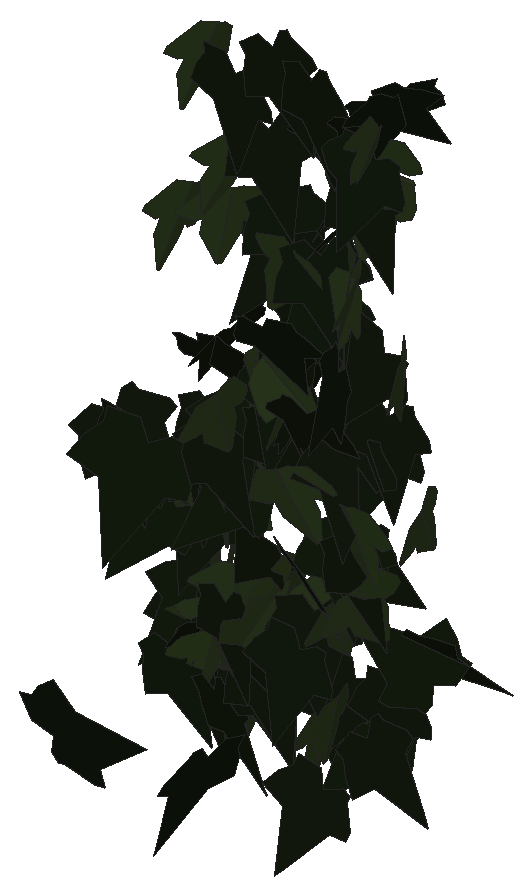
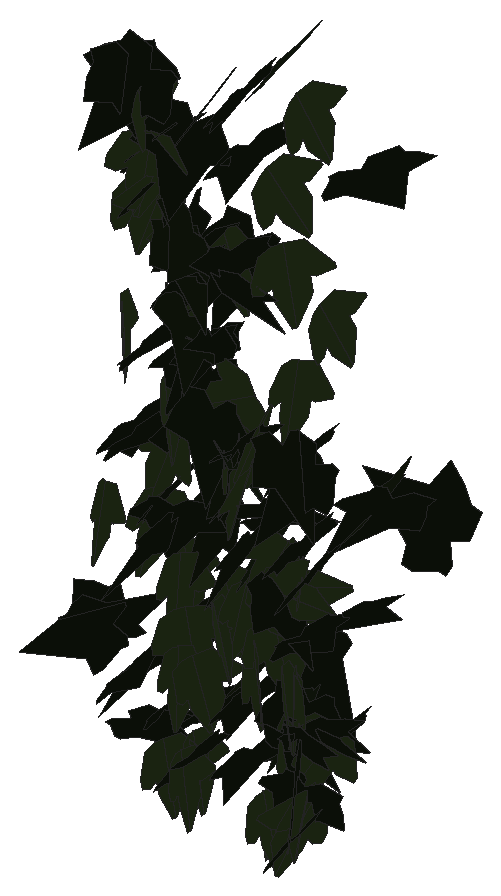
# SketchUp Ruby script. Lengths in inches.
U = 1.inch
M = Sketchup.active_model
def pt(a) = Geom::Point3d.new(a.map { |v| v * U })
def face(e, loops, mat)
  f = e.add_face(loops[0].map { |a| pt(a) })
  loops[1..].each { |l| e.add_face(l.map { |a| pt(a) }).erase! }
  f.material = f.back_material = mat if mat
  f
end
# faces: each face lists its corners as indices into pts; further lists are holes
def faces(e, pts, list, mat = nil) = list.each { |f| face(e, (f[0].is_a?(Array) ? f : [f]).map { |l| l.map { |i| pts[i] } }, mat) }
# xy, xz, yz: faces in a plane at the given z, y or x. An outline is a flat list of corners, or four numbers for a rectangle; further outlines are holes
def ring(l) = l.size == 4 ? [[l[0], l[1]], [l[2], l[1]], [l[2], l[3]], [l[0], l[3]]] : l.each_slice(2).to_a
def flat(e, list, mat, &to3) = list.each { |f| face(e, (f[0].is_a?(Array) ? f : [f]).map { |l| ring(l).map { |u, v| to3.(u, v) } }, mat) }
def xy(e, z, list, mat = nil) = flat(e, list, mat) { |x, y| [x, y, z] }
def xz(e, y, list, mat = nil) = flat(e, list, mat) { |x, z| [x, y, z] }
def yz(e, x, list, mat = nil) = flat(e, list, mat) { |y, z| [x, y, z] }
def lines(e, pts, list) = list.each { |a, b| e.add_line(pt(pts[a]), pt(pts[b])) }
# prism: a flat outline (further loops are holes) pulled along v
def prism(e, loops, v, mat = nil)
  f = face(e, loops, mat); d = Geom::Vector3d.new(v.map { |x| x * U })
  f.pushpull(f.normal.samedirection?(d) ? d.length : -d.length)
end
def box(e, o, s, mat = nil) = prism(e, [[o, [o[0] + s[0], o[1], o[2]], [o[0] + s[0], o[1] + s[1], o[2]], [o[0], o[1] + s[1], o[2]]]], [0, 0, s[2]], mat)
def at(x, y, z, deg = 0) = Geom::Transformation.translation(pt([x, y, z])) * Geom::Transformation.rotation(ORIGIN, Z_AXIS, deg.degrees)
def axes(o, x, y, z) = Geom::Transformation.new([*x, 0, *y, 0, *z, 0, *pt(o).to_a, 1])
def part(name) = M.definitions.add(name)
# library, detail: a bought-in or finely detailed component or shape, given as its bounding box
def library(name, o, s) = part(name).tap { |d| box(d.entities, o, s) }
def detail(e, o, s) = box(e.add_group.entities, o, s)
def put(e, d, t, mat = nil) = e.add_instance(d, t).tap { |i| i.material = mat if mat }
def group(e, t, mat = nil) = e.add_group.tap { |g| g.transformation = t; g.material = mat if mat }.entities
root = M.entities
M.materials.add("efeu1").color = [18, 25, 13]
M.materials.add("efeu2").color = [43, 57, 29]
c1 = part("ivyleaf_9")
p = [[1.54,2.16,1.25],[1.36,2.04,1.19],[-0.21,0.99,0.68],[-0.71,1.11,0.82],[-0.85,0.86,0.67],[-0.8,0.17,0.21],
  [-0.9,-0.01,0.1],[-0.67,-0.16,-0.02],[-0.08,-0.08,-0.05],[-0.03,-0.6,-0.4],[0.65,-0.88,-0.66],[0.83,-0.6,-0.49],
  [1.29,-0.42,-0.43],[1.8125,-0.07,-0.26],[1.21,0.44,0.15]]
faces(c1.entities,p,[[0,1,2,3,4,5,6,7,8,9,10,11,12,13,14]],"efeu1")
c2 = part("ivyleaf_10")
p = [[0,0.5,-0.03],[-0.0625,2.02,-0.43],[-0.19,2.01,-0.46],[-0.54,1.05,-0.29],[-0.52,0.625,-0.18],[-0.83,0.76,-0.28],
  [-1.16,0.64,-0.33],[-1.15,0.33,-0.24],[-0.77,-0.39,0.02],[-0.3,-0.51,0.16],[0.04,-0.48,0.23],[-0.02,2.01,-0.4375],
  [-0.06,2.01,-0.43],[0.04,-0.49,0.23],[0.67,-0.49,0.14],[1.38,0.36,-0.2],[1.375,0.51,-0.24],[0.81,0.65,-0.19],
  [0.62,0.59,-0.15],[0.6,1.09,-0.28],[0.5,1.23,-0.31]]
faces(c2.entities,p,[[0,1,2,3,4,5,6,7,8,9,10],[11,12,0,13,14,15,16,17,18,19,20]],"efeu2")
put(root,c1,axes([540.38,125.45,283.63],[-0.65075,-0.88361,0.42411],[-0.08524,-0.45613,-1.08111],[0.97641,-0.62872,0.18828]))
put(root,c2,axes([540.41,127.79,277.28],[-0.22429,1.09547,0.15556],[-0.17,0.12272,-1.10932],[-1.09332,-0.24382,0.14058]))
put(root,c1,axes([540.71,127.25,279.7],[-0.81743,-0.74221,0.3045],[-0.15597,-0.27939,-1.09973],[0.78694,-0.82635,0.09833]))
put(root,c1,axes([539.93,123.5625,287.6],[0.12835,-0.81486,-0.97339],[0.31526,0.96816,-0.76891],[1.22967,-0.16316,0.29873]))
put(root,c1,axes([540.91,127.39,278.66],[0.33903,-0.18207,-1.08033],[-0.99643,0.41884,-0.38329],[0.45541,1.05196,-0.03437]))
put(root,c2,axes([540.39,127.84,276.75],[0.49453,0.88418,0.52386],[0.02272,0.5718,-0.98655],[-1.02746,0.43821,0.23032]))
put(root,c1,axes([540.28,127.875,277.89],[-0.50158,-0.50398,-0.88565],[0.63375,0.61871,-0.711],[0.79796,-0.80818,0.00798]))
put(root,c2,axes([540.5,126.39,279.03],[-0.93713,-0.3643,-0.56454],[0.54156,0.16389,-1.00473],[0.39766,-1.08169,0.0379]))
put(root,c1,axes([540.65,126.93,279.63],[-0.86891,-0.55862,-0.51625],[0.58346,0.01334,-0.99648],[0.488,-1.01061,0.2722]))
put(root,c1,axes([540.44,128.06,276.05],[0.24819,-1.10286,-0.01708],[-0.01702,0.01368,-1.13036],[1.10286,0.2484,-0.0136]))
put(root,c1,axes([541.4375,127.43,279.43],[-1.09529,-0.30009,-0.15658],[0.1501,0.0447,-1.13565],[0.30339,-1.10552,-0.00342]))
put(root,c2,axes([541.18,125.4375,295.29],[-0.05817,-1.0711,0.57084],[0.15103,-0.57344,-1.06059],[1.20428,0.02018,0.16058]))
put(root,c1,axes([540.62,123.45,287.15],[0.26578,-1.1366,0.50822],[0.22263,-0.46791,-1.16288],[1.22499,0.33164,0.10108]))
put(root,c1,axes([541.14,126.9375,283.3],[-0.39388,-1.0784,0.22297],[-0.00482,-0.23511,-1.14565],[1.1012,-0.38676,0.07474]))
put(root,c2,axes([541.33,126.98,281.04],[0.7886,-0.85793,-0.05577],[0.20666,0.26262,-1.11775],[0.83453,0.74567,0.32949]))
put(root,c1,axes([541,125.04,278.53],[0.44245,-1.02896,-0.33743],[-0.05946,0.34087,-1.11743],[1.08124,0.4398,0.07663]))
put(root,c2,axes([541.6875,126.27,278.76],[-0.3156,-1.0866,0.26717],[0.06648,-0.29532,-1.12252],[1.11698,-0.28944,0.1423]))
put(root,c1,axes([541.34,126.17,289.6],[1.10842,0.35329,-0.13884],[-0.15449,0.02844,-1.16103],[-0.34673,1.11671,0.0735]))
put(root,c1,axes([541.31,126.65,285.27],[0.08848,-1.11835,0.33834],[-0.00158,-0.33942,-1.12151],[1.16841,0.08423,-0.02714]))
put(root,c1,axes([541.91,125.64,279.64],[0.31079,1.09986,-0.06636],[-0.02036,-0.06321,-1.14292],[-1.10167,0.31145,0.0024]))
put(root,c2,axes([542.52,125.75,284.13],[0.37256,0.18084,1.13241],[-1.04788,-0.42999,0.41342],[0.46584,-1.11187,0.0243]))
put(root,c2,axes([542.3,127.08,284.67],[-0.2639,-0.39551,1.06163],[-0.58514,-0.88582,-0.47547],[0.9701,-0.64189,0.00201]))
put(root,c1,axes([542.1875,126.64,290.23],[-0.32154,1.09711,-0.29601],[0.02419,-0.30096,-1.14171],[-1.13608,-0.31692,0.05947]))
put(root,c2,axes([541.78,127.01,281.19],[0.49372,-1.03052,-0.18486],[0.02567,0.21624,-1.13688],[1.04666,0.4808,0.11509]))
put(root,c1,axes([541.37,126.7,286.83],[0.23385,-1.144,-0.19589],[-0.05405,0.18888,-1.16756],[1.15939,0.23955,-0.01492]))
put(root,c1,axes([542.3,126.9375,284.94],[-0.40227,0.92276,-0.5849],[0.26608,-0.52177,-1.00617],[-1.05962,-0.48134,-0.03061]))
put(root,c2,axes([541.96,127.11,276.15],[-0.75196,0.84847,-0.21901],[0.13637,-0.17177,-1.13367],[-0.8656,-0.76413,0.01166]))
put(root,c2,axes([542.375,127.3,276.15],[-0.18217,-1.12207,0.06098],[-0.00762,-0.06054,-1.13675],[1.1237,-0.18231,0.00218]))
put(root,c2,axes([542.3,125.79,285.2],[-0.82077,0.76875,-0.31185],[0.11634,-0.32768,-1.114],[-0.8214,-0.81458,0.15382]))
put(root,c2,axes([542.51,125.6875,279.6875],[-0.5135,1.01183,0.15132],[-0.09164,0.12315,-1.13438],[-1.01897,-0.52098,0.02576]))
put(root,c2,axes([543.12,124.32,302.45],[-0.12069,-1.12356,0.51681],[0.06712,-0.52445,-1.12449],[1.2349,-0.0813,0.11163]))
put(root,c2,axes([542.89,126.13,285.58],[-1.09129,0.19974,-0.3925],[0.39047,-0.04621,-1.10918],[-0.20367,-1.15881,-0.02342]))
put(root,c2,axes([543.44,125.52,281.86],[-0.84232,-0.73608,0.27744],[-0.1437,-0.25565,-1.11458],[0.77339,-0.84919,0.09506]))
put(root,c2,axes([543.81,126.41,280.93],[-0.57369,0.39819,0.94383],[-0.86003,0.40048,-0.69171],[-0.55653,-1.02935,0.09599]))
put(root,c1,axes([543.33,126.35,287.47],[-0.85193,-0.82503,0.11182],[0.09268,-0.25297,-1.16034],[0.8274,-0.82116,0.24511]))
put(root,c2,axes([543.64,124.74,296.38],[-0.68544,-0.99741,0.17976],[-0.03196,-0.19564,-1.20734],[1.01297,-0.68108,0.08355]))
put(root,c1,axes([543.52,126.9,286.32],[0.50258,-0.84126,-0.63918],[-0.27987,0.57652,-0.97885],[1.01879,0.57338,0.04641]))
put(root,c1,axes([543.49,126.78,277.8],[0.15118,-1.04498,-0.44736],[-0.0214,0.4486,-1.05511],[1.13651,0.14745,0.03964]))
put(root,c2,axes([543.84,126.73,288.89],[-0.36046,0.81326,0.77222],[0.3253,-0.70043,0.8895],[1.07326,0.48543,-0.01025]))
put(root,c1,axes([543.32,124.51,277.92],[0.80571,-0.96704,0.02435],[0.01613,-0.01825,-1.2587],[0.96721,0.80587,0.00071]))
put(root,c2,axes([543.97,126.7,288.34],[-0.36398,1.11877,0.07061],[-0.02641,0.06566,-1.17648],[-1.12068,-0.36491,0.00479]))
put(root,c1,axes([544.36,124.78,285.97],[-0.86593,-0.65817,0.41688],[-0.15052,-0.47021,-1.05502],[0.76441,-0.83817,0.26451]))
put(root,c2,axes([544.56,124.07,298.9],[-0.26116,-1.05133,0.58337],[-0.12424,-0.57019,-1.08318],[1.19591,-0.28882,0.01487]))
put(root,c1,axes([543.88,123.34,288.16],[0.44528,-1.04105,-0.37356],[0.00583,0.4049,-1.12144],[1.10603,0.41698,0.15631]))
put(root,c1,axes([544,124.15,281.61],[0.39263,-1.09628,0.11826],[0.03322,-0.11372,-1.16445],[1.10214,0.39397,-0.00703]))
put(root,c1,axes([544.5625,126.46,289.29],[-0.16553,-1.16069,0.13177],[-0.02651,-0.12932,-1.17241],[1.16785,-0.16745,-0.00793]))
put(root,c1,axes([544.28,124.4,280.68],[0.76311,-0.82894,-0.30772],[-0.09695,0.32558,-1.11748],[0.87888,0.75566,0.14392]))
put(root,c2,axes([544.9,126.83,282.58],[0.47049,-1.0577,-0.09463],[-0.01483,0.09695,-1.15734],[1.06183,0.47002,0.02576]))
put(root,c2,axes([544.9375,122.45,290.25],[-0.24079,-1.11207,-0.41383],[0.1231,0.39658,-1.13732],[1.18017,-0.26826,0.0342]))
put(root,c2,axes([544.99,126.11,288.57],[0.36451,-1.07837,-0.26785],[0.02805,0.29074,-1.13234],[1.11078,0.34654,0.11649]))
put(root,c1,axes([544.55,125.92,287.73],[0.41052,-1.10678,-0.05108],[-0.02237,0.04619,-1.18045],[1.10773,0.4111,-0.0049]))
put(root,c1,axes([544.7,125.07,284.01],[-0.20906,-0.73732,0.96269],[0.15922,-0.98512,-0.71993],[1.2021,0.00225,0.26278]))
put(root,c1,axes([544.62,125.39,279.14],[0.18519,-1.16517,-0.30096],[0.02532,0.30821,-1.17765],[1.20315,0.17286,0.07111]))
put(root,c2,axes([545.125,125.2,282.55],[-0.13908,-1.01817,-0.53863],[0.14681,0.52245,-1.02549],[1.14247,-0.19108,0.06621]))
put(root,c2,axes([544.96,123.96,280.65],[-0.20797,-1.05143,0.59792],[0.09845,0.58997,1.07169],[-1.20554,0.22956,-0.01563]))
put(root,c1,axes([545.79,125.7,289.13],[-0.95993,0.67363,-0.119],[0.0906,-0.07804,-1.17265],[-0.67804,-0.96412,0.01177]))
put(root,c1,axes([545.55,126.4,290.4],[0.07875,1.18539,0.08268],[0.00058,0.08282,-1.18799],[-1.18827,0.0786,0.0049]))
put(root,c1,axes([545.68,125.62,295.32],[-1.1551,-0.31213,-0.1349],[0.15283,-0.04986,-1.19333],[0.30375,-1.16188,0.08745]))
put(root,c2,axes([545.45,128.09,277.05],[0.07837,-1.1181,-0.11985],[0.01628,0.12126,-1.12057],[1.12438,0.07618,0.02458]))
put(root,c2,axes([545.49,125.51,282.86],[-0.03318,-1.14737,0.18508],[0.01832,-0.18565,-1.14761],[1.16205,-0.02984,0.02338]))
put(root,c1,axes([544.27,115.01,280.88],[0.3837,-0.27467,1.40411],[1.17468,-0.76942,-0.47152],[0.81676,1.23562,0.01851]))
put(root,c1,axes([544.72,126.58,288.32],[0.4548,-0.0989,-1.08639],[1.04312,-0.30502,0.46446],[-0.31923,-1.13756,-0.03009]))
put(root,c1,axes([545.28,128.05,277.46],[0.10346,-1.12618,-0.01265],[-0.00402,0.01234,-1.13092],[1.12624,0.1035,-0.00287]))
put(root,c2,axes([545.83,126.92,280.19],[-0.48709,-1.02703,0.27994],[0.0071,-0.31098,-1.12857],[1.06448,-0.46788,0.13562]))
put(root,c1,axes([546.1,120.45,278.18],[-0.38406,0.96601,-0.88686],[0.33952,-0.81936,-1.03951],[-1.26666,-0.51252,-0.00973]))
put(root,c2,axes([545.93,126.77,277.05],[0.0938,-1.14469,-0.13274],[0.00078,0.13324,-1.14846],[1.15236,0.09309,0.01158]))
put(root,c1,axes([545.49,125.49,296.4],[-0.03595,-1.03805,-0.60014],[0.07048,0.59755,-1.03778],[1.19698,-0.06636,0.04308]))
put(root,c1,axes([545.53,124.73,302.58],[0.46175,-1.11229,-0.30252],[-0.0624,0.30129,-1.20302],[1.151,0.46255,0.05614]))
put(root,c2,axes([546.26,128.09,277.23],[-0.3191,-1.08053,0.06525],[-0.00791,-0.0657,-1.12661],[1.08247,-0.31901,0.01101]))
put(root,c2,axes([546.23,127.39,280.58],[-0.11598,-1.09817,-0.32836],[0.02213,0.32783,-1.10421],[1.14599,-0.11747,-0.01191]))
put(root,c1,axes([545.56,122.63,302.59],[0.12955,-1.19611,0.4608],[0.17151,-0.4428,-1.19763],[1.27028,0.18177,0.1147]))
put(root,c1,axes([545.8,124.11,299.9],[0.1137,-1.16031,-0.39927],[-0.04906,0.39636,-1.16583],[1.22611,0.12346,-0.00962]))
put(root,c2,axes([545.31,124.88,290.46],[0.56116,0.12187,1.09187],[1.07516,0.19124,-0.57392],[-0.22596,1.21264,-0.01922]))
put(root,c1,axes([545.96,126.01,292.99],[0.29745,-0.78401,-0.84788],[-0.27472,0.80237,-0.83831],[1.12165,0.40444,0.01952]))
put(root,c2,axes([546.41,126.75,281.82],[-0.83727,-0.80292,0.19809],[0.04109,-0.32193,-1.1312],[0.82597,-0.79789,0.25707]))
put(root,c2,axes([546.91,124.03,295.48],[-1.03074,-0.03764,0.63935],[-0.6321,-0.13529,-1.02702],[0.10314,-1.20536,0.0953]))
put(root,c1,axes([546.87,126.125,293.55],[-0.13015,1.01193,0.63516],[-0.12921,0.62325,-1.01943],[-1.18774,-0.17869,0.0413]))
put(root,c1,axes([547.11,125.65,296.6875],[0.0873,0.75209,0.94289],[-0.06813,0.94692,-0.749],[-1.20418,0.00095,0.11074]))
put(root,c1,axes([546.41,126.19,292.77],[-0.0048,-1.05681,-0.56667],[0.06233,0.56569,-1.05551],[1.19753,-0.03368,0.05266]))
put(root,c1,axes([547.49,125.71,296.32],[-0.34227,1.1467,0.01347],[-0.08186,-0.01041,-1.19392],[-1.14386,-0.34238,0.08141]))
put(root,c1,axes([546.67,125.41,281.63],[-0.21887,-1.12441,-0.29998],[0.09549,0.28686,-1.14489],[1.15981,-0.23581,0.03766]))
put(root,c1,axes([546.99,127.02,278.6],[-0.23698,-0.98415,0.52069],[-0.02206,-0.5281,-1.00819],[1.11318,-0.21998,0.09087]))
put(root,c1,axes([547.58,123.875,290.1],[0.7957,0.51951,-0.76299],[-0.69996,-0.3171,-0.94588],[-0.60175,1.05581,0.09134]))
put(root,c2,axes([547.5,126.41,290.45],[0.33165,-1.07137,-0.3998],[-0.09849,0.38797,-1.12136],[1.13929,0.34542,0.01945]))
put(root,c1,axes([546.86,125.03,301.69],[0.44536,-1.1524,0.09873],[-0.00185,-0.10651,-1.23482],[1.15662,0.44357,-0.04]))
put(root,c1,axes([547.03,125.74,295.16],[0.11149,-1.18236,-0.20142],[-0.0325,0.19924,-1.18753],[1.19896,0.11535,-0.01346]))
put(root,c2,axes([547.29,123.14,287.86],[-1.14292,-0.2646,-0.40805],[0.40058,0.07879,-1.17308],[0.27579,-1.21101,0.01284]))
put(root,c1,axes([547.6,124.98,300.46],[0.88976,0.76933,-0.3742],[-0.36009,-0.15296,-1.17069],[-0.77603,0.95305,0.11418]))
put(root,c1,axes([547.36,123.37,284.74],[1.1538,-0.1851,-0.55266],[-0.54116,0.11494,-1.16829],[0.21643,1.27416,0.0251]))
put(root,c1,axes([547.48,123.54,281.34],[-0.24426,-1.11693,0.32571],[0.01897,-0.33659,-1.14001],[1.16329,-0.22904,0.08698]))
put(root,c1,axes([547.71,121.54,294.36],[1.06649,0.46332,-0.34294],[-0.30372,-0.16134,-1.1625],[-0.48993,1.10859,-0.02586]))
put(root,c1,axes([547.59,124.59,295.62],[-0.01758,-1.11727,-0.50146],[0.02046,0.50117,-1.11735],[1.22447,-0.02441,0.01147]))
put(root,c2,axes([548.04,125.08,282.64],[-0.11779,-1.13347,-0.34215],[0.07707,0.33577,-1.13886],[1.18147,-0.13491,0.04018]))
put(root,c1,axes([548.48,127.06,277.41],[-0.95066,-0.6272,0.21778],[-0.14349,-0.17728,-1.1369],[0.64824,-0.95904,0.06773]))
put(root,c1,axes([548.375,123.6,276.42],[-0.46966,-0.98914,0.37014],[-0.08336,-0.3691,-1.09215],[1.05283,-0.47047,0.07864]))
put(root,c1,axes([548.2,125.21,285.14],[-0.5879,-0.80601,-0.62732],[0.43303,0.45885,-0.99537],[0.92503,-0.72706,0.06726]))
put(root,c2,axes([548.51,124.9,295.39],[0.71061,-0.9389,-0.27094],[-0.00583,0.33092,-1.16205],[0.9772,0.68473,0.19009]))
put(root,c1,axes([548.38,125.42,284.4375],[0.58303,-0.41374,-0.93092],[-0.38984,0.90034,-0.6443],[0.94118,0.62923,0.3098]))
put(root,c2,axes([548.5,125.69,297.87],[0.38066,1.0859,0.39605],[0.01083,0.41361,-1.14445],[-1.15582,0.36151,0.11971]))
put(root,c2,axes([548.84,125.98,299.58],[-1.17382,-0.28732,0.00456],[-0.00676,0.00845,-1.20844],[0.28727,-1.1738,-0.00982]))
put(root,c1,axes([548.65,114.09,293.58],[-0.6693,-1.27237,0.04912],[-0.00068,-0.05514,-1.43745],[1.27332,-0.66883,0.02506]))
put(root,c1,axes([548.58,124.91,288.52],[-0.35496,-1.13337,-0.22129],[0.07493,0.20841,-1.18762],[1.15233,-0.36267,0.00906]))
put(root,c2,axes([549.03,126.07,297.91],[-0.61969,-0.94713,0.40045],[-0.05124,-0.43852,-1.11647],[1.02703,-0.59336,0.18592]))
put(root,c1,axes([548.85,126.15,291.8],[-0.3611,-0.96355,0.6098],[-0.06576,-0.62099,-1.02016],[1.1384,-0.3415,0.1345]))
put(root,c1,axes([548.53,125.625,298.18],[0.25058,-1.157,-0.28827],[0.00041,0.29465,-1.18225],[1.19237,0.24305,0.06099]))
put(root,c1,axes([548.8,126.73,288.55],[-0.30054,-1.07879,0.36576],[0.00377,-0.37921,-1.11538],[1.1391,-0.28337,0.1002]))
put(root,c2,axes([549.06,124.12,295.05],[1.03634,-0.5924,-0.11984],[-0.06299,0.13072,-1.1909],[0.60111,1.03503,0.08182]))
put(root,c2,axes([549.12,123.6875,292.33],[0.46941,-1.00167,-0.43361],[0.01682,0.47859,-1.08737],[1.09137,0.42345,0.20326]))
put(root,c1,axes([548.75,126.71,289.09],[-0.00297,-1.17707,-0.08101],[-0.00043,0.08101,-1.17707],[1.17985,-0.00293,-0.00064]))
put(root,c2,axes([549.29,124.11,295.42],[0.50746,-1.07227,-0.18734],[-0.09364,0.16292,-1.18619],[1.08447,0.51581,-0.01476]))
put(root,c1,axes([549.06,125.43,299.4],[-0.33868,-1.09804,0.41733],[-0.00425,-0.43318,-1.14319],[1.17466,-0.31815,0.11619]))
put(root,c2,axes([549.34,125.33,300.87],[0.21777,-1.1235,0.44119],[0.09166,-0.43162,-1.14439],[1.20353,0.23617,0.00733]))
put(root,c1,axes([549.16,126.57,278.94],[-0.04358,-1.14776,0.22142],[-0.01392,-0.22105,-1.14858],[1.16884,-0.04543,-0.00542]))
put(root,c2,axes([549.45,123.98,286.75],[-1.13143,0.26491,-0.24577],[0.22773,-0.10447,-1.16101],[-0.28057,-1.1531,0.04872]))
put(root,c1,axes([549.06,124.28,285.31],[0.47979,-1.0469,-0.22332],[-0.0635,0.21646,-1.15116],[1.06857,0.48293,0.03186]))
put(root,c2,axes([549.85,127.01,285.76],[0.16124,-0.95516,-0.63787],[0.00587,0.6448,-0.96406],[1.14856,0.1308,0.09448]))
put(root,c2,axes([549.82,123.95,284.11],[-0.38212,-1.06188,-0.52427],[0.23783,0.47085,-1.12703],[1.16012,-0.44629,0.05837]))
put(root,c1,axes([550.18,125.15,302.25],[0.10263,1.11082,-0.52236],[-0.04933,-0.52003,-1.11555],[-1.22651,0.11387,0.00116]))
put(root,c1,axes([550.68,126.42,280.14],[-0.16629,0.45298,1.04351],[-1.13628,-0.11656,-0.13048],[0.05439,-1.05023,0.46456]))
put(root,c1,axes([549.6,125.02,301.98],[0.95946,0.73595,0.21965],[0.19113,0.11164,-1.2089],[-0.74387,0.97793,-0.02729]))
put(root,c2,axes([550.19,121.95,280.93],[0.13538,-1.15524,-0.12506],[-0.01275,0.12442,-1.16315],[1.16192,0.13597,0.00181]))
put(root,c1,axes([549.78,124.41,278.42],[0.50014,-0.85881,-0.64286],[-0.11433,0.66258,-0.9741],[1.06665,0.4737,0.19702]))
put(root,c2,axes([550.32,125.34,292.28],[0.55441,-1.03296,-0.29326],[0.03443,0.34697,-1.15706],[1.07323,0.52247,0.18861]))
put(root,c1,axes([549.71,126.97,280.76],[1.05658,-0.05098,0.50818],[0.51034,0.05974,-1.05508],[0.01997,1.17092,0.07596]))
put(root,c1,axes([550.5,121.78,293.53],[0.13062,-0.31132,-1.225],[1.01255,-0.71132,0.28874],[-0.75649,-1.00584,0.17496]))
